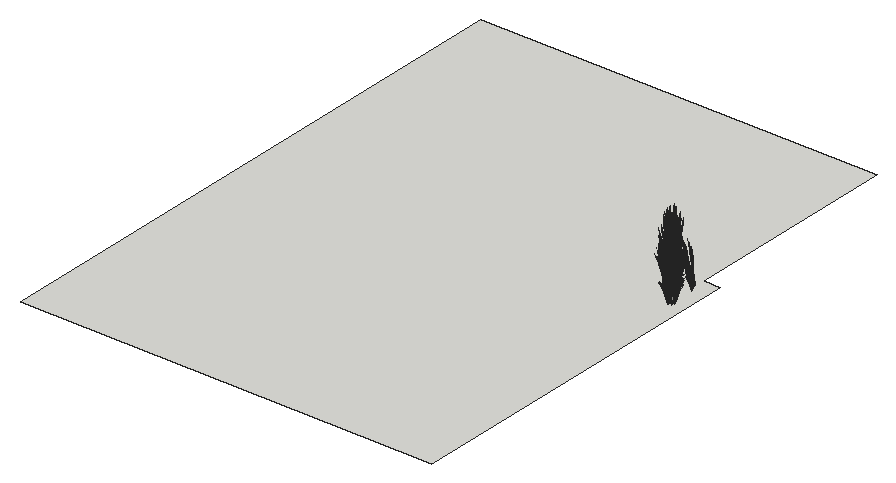
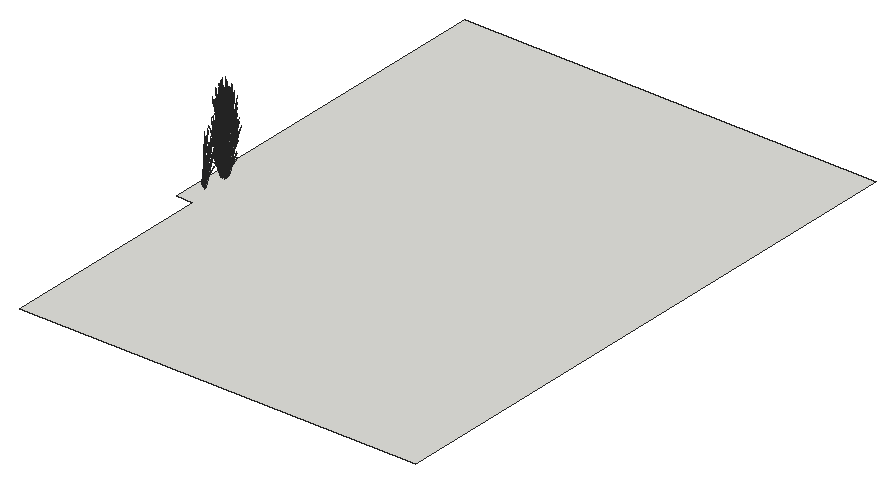
# SketchUp Ruby script. Lengths in inches.
U = 1.inch
M = Sketchup.active_model
def pt(a) = Geom::Point3d.new(a.map { |v| v * U })
def face(e, loops, mat)
  f = e.add_face(loops[0].map { |a| pt(a) })
  loops[1..].each { |l| e.add_face(l.map { |a| pt(a) }).erase! }
  f.material = f.back_material = mat if mat
  f
end
# faces: each face lists its corners as indices into pts; further lists are holes
def faces(e, pts, list, mat = nil) = list.each { |f| face(e, (f[0].is_a?(Array) ? f : [f]).map { |l| l.map { |i| pts[i] } }, mat) }
# xy, xz, yz: faces in a plane at the given z, y or x. An outline is a flat list of corners, or four numbers for a rectangle; further outlines are holes
def ring(l) = l.size == 4 ? [[l[0], l[1]], [l[2], l[1]], [l[2], l[3]], [l[0], l[3]]] : l.each_slice(2).to_a
def flat(e, list, mat, &to3) = list.each { |f| face(e, (f[0].is_a?(Array) ? f : [f]).map { |l| ring(l).map { |u, v| to3.(u, v) } }, mat) }
def xy(e, z, list, mat = nil) = flat(e, list, mat) { |x, y| [x, y, z] }
def xz(e, y, list, mat = nil) = flat(e, list, mat) { |x, z| [x, y, z] }
def yz(e, x, list, mat = nil) = flat(e, list, mat) { |y, z| [x, y, z] }
def lines(e, pts, list) = list.each { |a, b| e.add_line(pt(pts[a]), pt(pts[b])) }
# prism: a flat outline (further loops are holes) pulled along v
def prism(e, loops, v, mat = nil)
  f = face(e, loops, mat); d = Geom::Vector3d.new(v.map { |x| x * U })
  f.pushpull(f.normal.samedirection?(d) ? d.length : -d.length)
end
def box(e, o, s, mat = nil) = prism(e, [[o, [o[0] + s[0], o[1], o[2]], [o[0] + s[0], o[1] + s[1], o[2]], [o[0], o[1] + s[1], o[2]]]], [0, 0, s[2]], mat)
def at(x, y, z, deg = 0) = Geom::Transformation.translation(pt([x, y, z])) * Geom::Transformation.rotation(ORIGIN, Z_AXIS, deg.degrees)
def axes(o, x, y, z) = Geom::Transformation.new([*x, 0, *y, 0, *z, 0, *pt(o).to_a, 1])
def part(name) = M.definitions.add(name)
# library, detail: a bought-in or finely detailed component or shape, given as its bounding box
def library(name, o, s) = part(name).tap { |d| box(d.entities, o, s) }
def detail(e, o, s) = box(e.add_group.entities, o, s)
def put(e, d, t, mat = nil) = e.add_instance(d, t).tap { |i| i.material = mat if mat }
def group(e, t, mat = nil) = e.add_group.tap { |g| g.transformation = t; g.material = mat if mat }.entities
root = M.entities
M.materials.add("LightPink_Translucent").color = [144, 107, 117]
M.materials["LightPink_Translucent"].alpha = 0.75
c1 = part("blade")
p = [[2.15,0.21,22],[0,0.17,0],[0.09,0.45,0],[2.18,0.31,22],[2.29,0.31,22],[0.38,0.45,0],
  [2.48,0.24,33],[2.49,0.24,33],[2.48,0.22,33]]
faces(c1.entities,p,[[0,1,2,3],[4,5,2,3],[6,3,4,7],[8,0,3,6]])
c2 = part("seeds")
p = [[0.3,-0.1,1.38],[-0.01,-0.03,1.59],[-0.01,-0.03,0.03],[0.14,-0.07,-0.07],[0.29,-0.03,3],[0.15,0.01,3.11]]
faces(c2.entities,p,[[0,1,2,3],[1,0,4,5]],"LightPink_Translucent")
c3 = part("blade with seeds")
put(c3.entities,c1,at(0,0,0))
put(c3.entities,c2,axes([2.4,0.25,30.99],[1.5799,-0.05474,1.17369],[-0.12525,1.92788,0.29478],[-0.07173,-0.02425,1.56792]))
xy(root,1398,[[33.57,367.54,339.57,367.54,339.57,634.9,327.57,634.9,327.57,795.7,33.57,795.7]])
put(root,c3,axes([331.43,599.32,1402.73],[0.26007,-0.1585,0.0643],[0.12729,0.28902,0.50621],[-0.02512,-0.1274,0.77189]))
put(root,c3,axes([330.51,599.69,1402.98],[-0.30095,-0.22541,-0.71045],[0.21388,-0.395,0.08574],[-0.10904,-0.13459,1.00501]))
put(root,c3,axes([330.4,599.39,1402.53],[-0.05451,-0.37564,-0.35414],[0.31161,-0.09919,0.4572],[-0.0837,-0.10765,0.87481]))
put(root,c3,axes([330.54,599.36,1402.73],[0.16041,-0.29625,0.0643],[0.22843,0.17248,0.50621],[-0.07385,-0.09498,0.77189]))
put(root,c3,axes([329.92,599.32,1399.49],[-0.03419,0.06144,1.76342],[-0.3455,0.13246,-0.26939],[-0.08346,-0.12049,0.30037]))
put(root,c3,axes([330.49,601.01,1400.1],[-0.14494,-0.47823,-0.69835],[0.41752,-0.17223,-0.18329],[-0.01602,-0.16194,1.54149]))
put(root,c3,axes([329.73,599.94,1401.875],[0.1311,0.08035,1.71376],[-0.27131,0.33708,0.13857],[-0.16909,-0.15206,0.73262]))
put(root,c3,axes([332.43,599.55,1399.49],[-0.05283,-0.03674,1.76342],[-0.13569,-0.41045,-0.26939],[0.09154,-0.11138,0.30037]))
put(root,c3,axes([331.33,599.64,1403.05],[-0.1064,0.35863,0.35414],[-0.31043,-0.1046,-0.4572],[-0.02846,-0.14439,0.87481]))
put(root,c3,axes([330.37,599.7,1402.68],[-0.34827,0.11086,-0.51099],[-0.06092,-0.41983,-0.3958],[-0.09354,-0.12031,0.97773]))
put(root,c3,axes([332.125,599.79,1402.73],[0.25132,0.3182,0.48003],[-0.2669,0.27442,0.3958],[0.04636,-0.14929,0.9933]))
put(root,c3,axes([330.61,599.33,1403.43],[-0.23555,0.44708,-0.13619],[-0.34112,-0.25757,-0.75594],[-0.11858,-0.12631,1.14864]))
put(root,c3,axes([332.22,599.82,1402.73],[0.29004,0.02173,0.0643],[-0.00795,0.32812,0.50621],[0.03035,-0.12569,0.77189]))
put(root,c3,axes([332,600.04,1403.05],[-0.23881,0.24554,0.35414],[-0.22606,-0.28036,-0.4572],[0.0344,-0.14245,0.87481]))
put(root,c3,axes([332.42,600.71,1402.98],[0.18436,-0.36797,-0.71045],[0.32306,0.26151,0.08574],[0.11008,-0.13332,1.00501]))
put(root,c3,axes([330.43,599.63,1400.375],[-0.22066,-0.46731,0],[0.36918,-0.26061,-0.51607],[0.08408,-0.05936,1.63711]))
put(root,c3,axes([332.41,600.53,1402.68],[-0.09067,-0.42583,-0.51099],[0.34336,-0.07449,-0.3958],[0.0984,-0.11438,0.97773]))
put(root,c3,axes([330.92,599.07,1400.13],[-0.2439,0.26754,-0.03893],[-0.22348,-0.29302,-0.17649],[-0.01573,-0.08303,0.58215]))
put(root,c3,axes([329.71,599.2,1402.72],[-0.07594,-0.00329,1.74944],[-0.24177,0.32918,-0.27667],[-0.129,-0.06726,0.14031]))
put(root,c3,axes([332.58,600.84,1403.03],[-0.32648,-0.25715,-0.1216],[0.18809,-0.3724,-0.67495],[0.09224,-0.12945,1.02557]))
put(root,c3,axes([331.23,602.24,1401.33],[0.305,0.18805,1.51261],[-0.29879,0.40513,0.59816],[-0.13384,-0.24012,1.26806]))
put(root,c3,axes([330.59,599.7,1403.05],[0.05451,0.37564,0.35414],[-0.31161,0.09919,-0.4572],[-0.0837,-0.10765,0.87481]))
put(root,c3,axes([329.63,600.94,1400.02],[0,-0.46636,-0.49651],[0.39487,0,0],[0,-0.10622,1.57504]))
put(root,c3,axes([330.73,599.5625,1400.02],[0.33032,-0.23318,-0.49651],[0.19744,0.41812,0],[0.07523,-0.05311,1.57504]))
put(root,c3,axes([332.69,600.37,1400.59],[-0.12609,-0.01381,1.43002],[-0.12917,-0.37055,-0.30754],[0.1549,-0.10482,0.61141]))
put(root,c3,axes([329.65,599.95,1403.09],[0.29147,-0.34417,0.53763],[0.25138,0.3655,0.4433],[-0.13675,-0.06349,1.11249]))
put(root,c3,axes([333.38,600.73,1402.71],[-0.0461,-0.00354,1.77383],[-0.19143,-0.37951,-0.16761],[0.07688,-0.12478,0.31391]))
put(root,c3,axes([331.12,600.52,1400.06],[0.23773,-0.35053,-0.62353],[0.29532,0.31785,-0.16365],[0.09526,-0.08744,1.37633]))
put(root,c3,axes([332.84,599.6875,1400.77],[-0.11756,0.2374,1.1486],[-0.10105,-0.31895,0.84392],[0.09709,-0.07992,0.25299]))
put(root,c3,axes([332.67,600.58,1402.53],[0.30722,-0.06665,-0.35414],[0.08112,0.381,0.4572],[0.08804,-0.10234,0.87481]))
put(root,c3,axes([329.78,599.94,1402.73],[0.01777,-0.35463,0.0643],[0.26836,0.00972,0.50621],[-0.1028,-0.03711,0.77189]))
put(root,c3,axes([330.71,601.13,1400.21],[0.17124,-0.42022,-0.44739],[0.35581,0.20224,0.21531],[0,-0.09687,1.43643]))
put(root,c3,axes([329.68,600.06,1402.53],[-0.20082,-0.29199,-0.35414],[0.2293,-0.2764,0.4572],[-0.1165,-0.04206,0.87481]))
put(root,c3,axes([330.86,600.93,1400.67],[-0.04113,-0.53214,-0.29095],[0.42835,-0.03218,-0.50002],[0.07543,-0.07088,1.59708]))
put(root,c3,axes([329.8,600.95,1400.03],[0.24637,-0.29097,-0.30978],[0.24637,0.29097,0.30978],[0,-0.09372,1.38974]))
put(root,c3,axes([329.7,599.56,1400.13],[-0.10181,0.3808,-0.03893],[-0.31336,-0.11714,-0.17649],[-0.04758,-0.06228,0.58215]))
put(root,c3,axes([332.42,600.8,1403.05],[-0.30722,0.06665,0.35414],[-0.08112,-0.381,-0.4572],[0.08804,-0.10234,0.87481]))
put(root,c3,axes([330.67,601.48,1400.67],[-0.39748,-0.22252,-0.29095],[0.19139,-0.46966,-0.50002],[-0.01249,-0.11531,1.59708]))
put(root,c3,axes([329.53,601.3,1400.375],[-0.44133,0,0],[0,-0.52122,-0.51607],[0,-0.11871,1.63711]))
put(root,c3,axes([329.61,600.37,1400.59],[0.06891,0.12984,1.43002],[-0.15879,0.35293,-0.30754],[-0.16304,-0.08436,0.61141]))
put(root,c3,axes([330.81,599.75,1400.03],[0.32928,0.11539,-0.30978],[-0.08291,0.40636,0.30978],[0.06638,-0.04686,1.38974]))
put(root,c3,axes([329.89,600.25,1402.98],[-0.35281,-0.01123,-0.71045],[0.0237,-0.47284,0.08574],[-0.14947,-0.0499,1.00501]))
put(root,c3,axes([332.7,600.74,1402.73],[0.2423,0.19613,0.0643],[-0.14107,0.2793,0.50621],[0.07768,-0.0903,0.77189]))
put(root,c3,axes([332.63,600.66,1402.73],[0.08753,0.42921,0.48003],[-0.34336,0.07449,0.3958],[0.1012,-0.10094,0.9933]))
put(root,c3,axes([333.55,601.18,1402.72],[0.04898,-0.07104,1.74944],[-0.06269,-0.43574,-0.27667],[0.12289,-0.08262,0.14031]))
put(root,c3,axes([329.875,601.16,1400.33],[-0.32829,0.39208,0.30756],[-0.32849,-0.38796,-0.36492],[-0.01146,-0.11134,1.64885]))
put(root,c3,axes([329.42,599.48,1402.71],[0.02617,0.04654,1.77383],[-0.12614,0.41836,-0.16761],[-0.12775,0.00303,0.31391]))
put(root,c3,axes([330.92,601.34,1400.43],[0.39767,0.22603,0.24065],[-0.19139,0.46966,0.50002],[0,-0.10827,1.60543]))
put(root,c3,axes([330.77,601.98,1400.4375],[0.09355,-0.55261,-0.23429],[0.44354,0.09633,0.51271],[-0.0775,-0.07631,1.5644]))
put(root,c3,axes([329.78,600.35,1402.68],[-0.25628,0.30892,-0.51099],[-0.22444,-0.32634,-0.3958],[-0.13021,-0.047,0.97773]))
put(root,c3,axes([329.97,600.21,1403.05],[0.20082,0.29199,0.35414],[-0.2293,0.2764,-0.4572],[-0.1165,-0.04206,0.87481]))
put(root,c3,axes([329.2,600.76,1400.77],[0.22533,-0.03337,1.1486],[-0.14293,0.29403,0.84392],[-0.11135,-0.04411,0.25299]))
put(root,c3,axes([330.79,601.03,1400.72],[-0.38326,0.02879,0.44739],[-0.03466,-0.47788,-0.21531],[0.06861,-0.04843,1.43643]))
put(root,c3,axes([329.91,600.02,1403.03],[-0.0189,0.47427,-0.1216],[-0.35781,-0.01296,-0.67495],[-0.13781,-0.03295,1.02557]))
put(root,c3,axes([329.8,601.375,1400.48],[0,0.46636,0.49651],[-0.39487,0,0],[0,-0.10622,1.57504]))
put(root,c3,axes([332.59,601.84,1403.03],[-0.17758,-0.42229,-0.1216],[0.31518,-0.20752,-0.67495],[0.13282,-0.05572,1.02557]))
put(root,c3,axes([332.57,601.48,1402.68],[0.09562,-0.42421,-0.51099],[0.32782,0.1454,-0.3958],[0.13199,-0.0389,0.97773]))
put(root,c3,axes([332.06,599.75,1400.375],[0.22066,-0.46731,0],[0.36918,0.26061,-0.51607],[0.08408,0.05936,1.63711]))
put(root,c3,axes([329.46,600.68,1401.875],[0.14639,-0.01056,1.71376],[-0.09712,0.45778,0.13857],[-0.20862,-0.02831,0.73262]))
put(root,c3,axes([330.73,601.75,1400.21],[-0.21202,-0.39143,-0.44739],[0.32115,-0.27564,0.21531],[-0.06861,-0.04843,1.43643]))
put(root,c3,axes([330.78,601.2,1400.36],[0.15345,0.52148,0.45755],[-0.43845,0.18134,0.17955],[0.00536,-0.09582,1.58856]))
put(root,c3,axes([332.92,601.6,1399.98],[-0.22732,0.05597,1.41583],[-0.03618,-0.44548,0.08104],[0.15921,-0.06743,0.80566]))
put(root,c3,axes([333.34,601.2,1400.26],[-0.21881,-0.29821,-0.06488],[0.23965,-0.27324,-0.29416],[0.0679,-0.01924,0.97024]))
put(root,c3,axes([330.7,601.61,1400.72],[-0.17124,0.42022,0.44739],[-0.35581,-0.20224,-0.21531],[0,-0.09687,1.43643]))
put(root,c3,axes([331.33,601.24,1400.21],[0,-0.53961,0],[0.44133,0,0],[0,0,1.79456]))
put(root,c3,axes([331.87,600,1400.48],[-0.33032,-0.23318,0.49651],[0.19744,-0.41812,0],[0.07523,0.05311,1.57504]))
put(root,c3,axes([332.51,601.63,1402.98],[0.31014,-0.20596,-0.71045],[0.17284,0.42397,0.08574],[0.14985,-0.04816,1.00501]))
put(root,c3,axes([330.54,601.9,1400.06],[-0.36714,-0.07646,-0.62353],[0.07747,-0.47163,-0.16365],[-0.10956,-0.05715,1.37633]))
put(root,c3,axes([331.12,600.9,1400.36],[-0.29264,0.42323,0.45755],[-0.34767,-0.3736,0.17955],[0.07055,-0.04224,1.58856]))
put(root,c3,axes([331.44,601.66,1400.3],[-0.32829,-0.4014,-0.06131],[0.32849,-0.40164,0],[-0.01146,-0.01402,1.75571]))
put(root,c3,axes([330.61,600.21,1400.47],[-0.10196,0.46348,0.17642],[-0.3731,-0.13116,0.35086],[0.06445,-0.00226,1.60407]))
put(root,c3,axes([332.47,601.72,1403.05],[-0.29332,-0.1301,0.35414],[0.08555,-0.37955,-0.4572],[0.11809,-0.0348,0.87481]))
put(root,c3,axes([329.4,601.02,1402.73],[0.09971,-0.42522,0.48003],[0.32782,0.1454,0.3958],[-0.12892,0.02555,0.9933]))
put(root,c3,axes([330.46,600.58,1399.59],[-0.3474,0.18671,1.28929],[-0.11057,-0.53572,0.50096],[0.21332,0.00891,1.46642]))
put(root,c3,axes([331.39,600.72,1400.62],[0.06809,-0.4162,0.1448],[0.33266,0.07225,-0.41347],[0.06054,0.04274,1.26744]))
put(root,c3,axes([329.37,600.91,1402.73],[-0.12963,-0.31798,0.0643],[0.23638,-0.15564,0.50621],[-0.1042,0.03071,0.77189]))
put(root,c3,axes([330.82,601.71,1400.36],[0.44609,0.09826,0.45755],[-0.09078,0.55493,0.17955],[-0.06519,-0.05359,1.58856]))
put(root,c3,axes([333.17,601.31,1399.49],[-0.01845,-0.0708,1.76342],[0.12793,-0.41416,-0.26939],[0.12905,-0.00596,0.30037]))
put(root,c3,axes([329.36,601.24,1399.49],[0.00895,0.0735,1.76342],[-0.18044,0.38382,-0.26939],[-0.12817,-0.01935,0.30037]))
put(root,c3,axes([331.25,600.83,1400.72],[-0.21202,-0.39143,0.44739],[0.32115,-0.27564,-0.21531],[0.06861,0.04843,1.43643]))
put(root,c3,axes([330.15,602.62,1400.03],[-0.08291,-0.40636,-0.30978],[0.32928,-0.11539,0.30978],[-0.06638,-0.04686,1.38974]))
put(root,c3,axes([330.58,602.6,1400.47],[0.37926,-0.12378,0.17642],[0.09365,0.46065,0.35086],[-0.03382,-0.06712,1.60407]))
put(root,c3,axes([331.36,600.86,1400.67],[0.35635,-0.30962,-0.29095],[0.23697,0.43749,-0.50002],[0.08792,0.04443,1.59708]))
put(root,c3,axes([332.78,601.67,1402.53],[0.29332,0.1301,-0.35414],[-0.08555,0.37955,0.4572],[0.11809,-0.0348,0.87481]))
put(root,c3,axes([330.0625,602.79,1400.02],[-0.33032,-0.23318,-0.49651],[0.19744,-0.41812,0],[-0.07523,-0.05311,1.57504]))
put(root,c3,axes([332.26,600.03,1400.02],[0.33032,0.23318,-0.49651],[-0.19744,0.41812,0],[0.07523,0.05311,1.57504]))
put(root,c3,axes([329.33,601.07,1402.53],[-0.29332,-0.1301,-0.35414],[0.08555,-0.37955,0.4572],[-0.11809,0.0348,0.87481]))
put(root,c3,axes([331.63,601.36,1400.21],[0.39487,0,0],[0,0.48281,0],[0,0,1.78407]))
put(root,c3,axes([330.96,601.97,1400.67],[-0.35635,0.30962,-0.29095],[-0.23697,-0.43749,-0.50002],[-0.08792,-0.04443,1.59708]))
put(root,c3,axes([331.74,600.23,1400.47],[-0.37926,0.12378,0.17642],[-0.09365,-0.46065,0.35086],[0.03382,0.06712,1.60407]))
put(root,c3,axes([331.98,601.2,1401.875],[-0.14639,0.01056,1.71376],[0.09712,-0.45778,0.13857],[0.20862,0.02831,0.73262]))
put(root,c3,axes([332.17,600.21,1400.03],[0.08291,0.40636,-0.30978],[-0.32928,0.11539,0.30978],[0.06638,0.04686,1.38974]))
put(root,c3,axes([332.73,601.83,1402.73],[0.12963,0.31798,0.0643],[-0.23638,0.15564,0.50621],[0.1042,-0.03071,0.77189]))
put(root,c3,axes([331.5,601.12,1400.38],[-0.44609,-0.09826,0.49198],[0.09078,-0.55493,0.19306],[0.06519,0.05359,1.70813]))
put(root,c3,axes([332.71,601.72,1402.73],[-0.09971,0.42522,0.48003],[-0.32782,-0.1454,0.3958],[0.12892,-0.02555,0.9933]))
put(root,c3,axes([331.15,602.49,1400.2],[-0.11516,-0.40207,0],[0.32884,-0.1408,0],[0,0,1.54371]))
put(root,c3,axes([330.93,602.11,1400.62],[-0.06809,0.4162,0.1448],[-0.33266,-0.07225,-0.41347],[-0.06054,-0.04274,1.26744]))
put(root,c3,axes([329.64,601.03,1403.05],[0.29332,0.1301,0.35414],[-0.08555,0.37955,-0.4572],[-0.11809,0.0348,0.87481]))
put(root,c3,axes([331.58,602.43,1400.18],[0.37054,-0.15823,-0.19198],[0.1302,0.45581,0.00008],[0.0409,-0.01749,1.73897]))
put(root,c3,axes([331.71,602.62,1400.47],[0.10196,-0.46348,0.17642],[0.3731,0.13116,0.35086],[-0.06445,0.00226,1.60407]))
put(root,c3,axes([331.62,601.57,1400.21],[0.24637,0.30123,0],[-0.24637,0.30123,0],[0,0,1.69266]))
put(root,c3,axes([330.22,601.01,1401.34],[0.10032,-0.06746,1.77064],[0.0346,0.47103,0.13857],[-0.2173,0.0625,0.63284]))
put(root,c3,axes([332.29,601.44,1400.47],[-0.2773,-0.3397,0.17642],[0.27945,-0.32949,0.35086],[-0.03063,0.06937,1.60407]))
put(root,c3,axes([331.78,600.93,1400.06],[0.36714,0.07646,-0.62353],[-0.07747,0.47163,-0.16365],[0.10956,0.05715,1.37633]))
put(root,c3,axes([333.4,601.75,1400.77],[-0.21807,0.07699,1.1486],[0.10265,-0.31819,0.84392],[0.11568,0.02177,0.25299]))
put(root,c3,axes([331.07,602.67,1400.2],[-0.35581,-0.20937,0],[0.17124,-0.43505,0],[0,0,1.62707]))
put(root,c3,axes([331.36,602.11,1400.46],[-0.34464,-0.37536,-0.25192],[0.29,-0.42149,0.5513],[-0.0928,0.04391,1.68216]))
put(root,c3,axes([330.45,602.83,1400.48],[0.33032,0.23318,0.49651],[-0.19744,0.41812,0],[-0.07523,-0.05311,1.57504]))
put(root,c3,axes([331.62,601.22,1400.72],[0.17124,-0.42022,0.44739],[0.35581,0.20224,-0.21531],[0,0.09687,1.43643]))
put(root,c3,axes([333.3,603.1,1402.71],[-0.03191,-0.04083,1.77383],[0.06981,-0.43764,-0.16761],[0.12571,-0.02796,0.31391]))
put(root,c3,axes([329.14,601.32,1402.72],[-0.05763,0.06055,1.74944],[0.0049,0.44239,-0.27667],[-0.13211,0.05753,0.14031]))
put(root,c3,axes([331.55,601.46,1400.29],[0,0.53934,-0.05637],[-0.44133,0,0],[0,0.01695,1.79368]))
put(root,c3,axes([329.53,601.26,1402.68],[-0.09562,0.42421,-0.51099],[-0.32782,-0.1454,-0.3958],[-0.13199,0.0389,0.97773]))
put(root,c3,axes([329.51,600.9,1403.03],[0.17758,0.42229,-0.1216],[-0.31518,0.20752,-0.67495],[-0.13282,0.05572,1.02557]))
put(root,c3,axes([331.58,601.08,1400.21],[0.21202,0.39143,-0.44739],[-0.32115,0.27564,0.21531],[0.06861,0.04843,1.43643]))
put(root,c3,axes([333.02,602.73,1401.93],[-0.06755,-0.39203,-0.03492],[0.31928,-0.09013,-0.15832],[0.06667,0.02485,0.52218]))
put(root,c3,axes([330.26,603.08,1400.375],[-0.22066,0.46731,0],[-0.36918,-0.26061,-0.51607],[-0.08408,-0.05936,1.63711]))
put(root,c3,axes([332.19,602.72,1403.03],[0.0189,-0.47427,-0.1216],[0.35781,0.01296,-0.67495],[0.13781,0.03295,1.02557]))
put(root,c3,axes([332.52,601.45,1400.48],[0,-0.46636,0.49651],[0.39487,0,0],[0,0.10622,1.57504]))
put(root,c3,axes([331.53,601.8,1400.72],[0.38326,-0.02879,0.44739],[0.03466,0.47788,-0.21531],[-0.06861,0.04843,1.43643]))
put(root,c3,axes([331.77,601.31,1400.62],[0.32884,-0.136,0.1448],[0.11516,0.38837,-0.41347],[0,0.08547,1.26744]))
put(root,c3,axes([332.14,602.53,1403.05],[-0.20082,-0.29199,0.35414],[0.2293,-0.2764,-0.4572],[0.1165,0.04206,0.87481]))
put(root,c3,axes([331.1875,602.03,1400.21],[-0.38326,0.02879,-0.44739],[-0.03466,-0.47788,0.21531],[-0.06861,0.04843,1.43643]))
put(root,c3,axes([332.99,602.26,1400.59],[-0.085,-0.1147,1.43002],[0.1106,-0.37943,-0.30754],[0.17198,0.0514,0.61141]))
put(root,c3,axes([331.47,602.68,1400.2],[0.35581,0.20937,0],[-0.17124,0.43505,0],[0,0,1.74954]))
put(root,c3,axes([332.5,602.44,1402.72],[0.07571,-0.00789,1.74944],[0.20767,-0.36231,-0.27667],[0.13467,0.04783,0.14031]))
put(root,c3,axes([331.61,603.14,1400.19],[-0.21791,-0.46895,-0.05142],[0.36918,-0.26061,0.51607],[-0.09097,0.04465,1.6363]))
put(root,c3,axes([331.53,602.01,1400.62],[0.26075,0.2802,0.1448],[-0.2175,0.31612,-0.41347],[-0.06054,0.04274,1.26744]))
put(root,c3,axes([329.47,602.08,1402.73],[-0.08753,-0.42921,0.48003],[0.34336,-0.07449,0.3958],[-0.1012,0.10094,0.9933]))
put(root,c3,axes([329.41,602,1402.73],[-0.2423,-0.19613,0.0643],[0.14107,-0.2793,0.50621],[-0.07768,0.0903,0.77189]))
put(root,c3,axes([329.52,601.48,1401.875],[0.12246,-0.09864,1.71376],[0.1031,0.45582,0.13857],[-0.19225,0.10302,0.73262]))
put(root,c3,axes([332.21,602.49,1402.98],[0.35281,0.01123,-0.71045],[-0.0237,0.47284,0.08574],[0.14947,0.0499,1.00501]))
put(root,c3,axes([331.8125,602.87,1400.48],[0.33032,-0.23318,0.49651],[0.19744,0.41812,0],[-0.07523,0.05311,1.57504]))
put(root,c3,axes([331.34,602.5,1400.29],[0.15345,0.53576,-0.06012],[-0.43845,0.18773,0],[0.00536,0.01871,1.72173]))
put(root,c3,axes([331.51,603.08,1400.03],[-0.32928,-0.11539,-0.30978],[0.08291,-0.40636,0.30978],[-0.06638,0.04686,1.38974]))
put(root,c3,axes([329.14,602.26,1400.59],[0.12266,0.03828,1.43002],[0.07906,0.39104,-0.30754],[-0.16661,0.0732,0.61141]))
put(root,c3,axes([329.6875,601.9375,1403.05],[0.30722,-0.06665,0.35414],[0.08112,0.381,-0.4572],[-0.08804,0.10234,0.87481]))
put(root,c3,axes([332.78,601.53,1400.375],[0.44133,0,0],[0,0.52122,-0.51607],[0,0.11871,1.63711]))
put(root,c3,axes([328.5,601.77,1402.71],[0.04504,0.01251,1.77383],[0.13934,0.41205,-0.16761],[-0.0922,0.10815,0.31391]))
put(root,c3,axes([332.61,601.8,1400.2],[-0.44111,-0.00373,-0.04976],[0,-0.52122,0.49943],[-0.01386,0.11865,1.58352]))
put(root,c3,axes([331.65,601.35,1400.67],[0.39748,0.22252,-0.29095],[-0.19139,0.46966,-0.50002],[0.01249,0.11531,1.59708]))
put(root,c3,axes([328.88,603.08,1400.77],[0.14709,-0.21136,1.1486],[0.05804,0.3346,0.84392],[-0.1063,0.05991,0.25299]))
put(root,c3,axes([332.42,602.6875,1402.53],[0.20082,0.29199,-0.35414],[-0.2293,0.2764,0.4572],[0.1165,0.04206,0.87481]))
put(root,c3,axes([332.52,601.875,1400.03],[-0.24637,0.29097,-0.30978],[-0.24637,-0.29097,0.30978],[0,0.09372,1.38974]))
put(root,c3,axes([331.46,601.9,1400.67],[0.04113,0.53214,-0.29095],[-0.42835,0.03218,-0.50002],[-0.07543,0.07088,1.59708]))
put(root,c3,axes([332.32,602.8,1402.73],[-0.01777,0.35463,0.0643],[-0.26836,-0.00972,0.50621],[0.1028,0.03711,0.77189]))
put(root,c3,axes([331.61,601.7,1400.21],[-0.17124,0.42022,-0.44739],[-0.35581,-0.20224,0.21531],[0,0.09687,1.43643]))
put(root,c3,axes([329.43,602.16,1402.53],[-0.30722,0.06665,-0.35414],[-0.08112,-0.381,0.4572],[-0.08804,0.10234,0.87481]))
put(root,c3,axes([332.34,602.6875,1402.73],[-0.26024,0.30729,0.48003],[-0.22444,-0.32634,0.3958],[0.1221,0.05668,0.9933]))
put(root,c3,axes([328.99,603.02,1403.65],[0.31145,0.12449,-0.06488],[-0.0958,0.38314,-0.29416],[-0.05094,0.05817,0.97024]))
put(root,c3,axes([331.2,602.31,1400.06],[-0.23773,0.35053,-0.62353],[-0.29532,-0.31785,-0.16365],[-0.09526,0.08744,1.37633]))
put(root,c3,axes([331.52,603.04,1403.05],[-0.05451,-0.37564,0.35414],[0.31161,-0.09919,-0.4572],[0.0837,0.10765,0.87481]))
put(root,c3,axes([331.62,602.9,1400.33],[0.44186,0.15158,0.30756],[-0.11054,0.54181,-0.36492],[-0.07313,0.06781,1.64885]))
put(root,c3,axes([331.59,603.27,1400.02],[-0.33032,0.23318,-0.49651],[-0.19744,-0.41812,0],[-0.07523,0.05311,1.57504]))
put(root,c3,axes([332.6875,601.89,1400.02],[0,0.46636,-0.49651],[-0.39487,0,0],[0,0.10622,1.57504]))
put(root,c3,axes([331.7,601.9375,1401.875],[-0.1311,-0.08035,1.71376],[0.27131,-0.33708,0.13857],[0.16909,0.15206,0.73262]))
put(root,c3,axes([331.72,600.88,1402.47],[-0.30498,-0.24231,1.38283],[0.32203,-0.37727,0.59665],[0.0984,0.22736,1.33663]))
put(root,c3,axes([329.53,601.9,1403.03],[0.32648,0.25715,-0.1216],[-0.18809,0.3724,-0.67495],[-0.09224,0.12945,1.02557]))
put(root,c3,axes([332.18,602.85,1400.77],[-0.19872,-0.13409,1.1486],[0.2566,-0.13625,0.84392],[0.06921,0.11541,0.25299]))
put(root,c3,axes([331.49,603.24,1403.03],[0.21031,-0.39918,-0.1216],[0.30457,0.22997,-0.67495],[0.10587,0.11278,1.02557]))
put(root,c3,axes([329.97,601.79,1401.875],[0.08815,-0.14329,1.71376],[0.22258,0.38678,0.13857],[-0.15267,0.17614,0.73262]))
put(root,c3,axes([329.6875,602.21,1402.68],[0.09067,0.42583,-0.51099],[-0.34336,0.07449,-0.3958],[-0.0984,0.11438,0.97773]))
put(root,c3,axes([330.1,602.7,1403.05],[0.23881,-0.24554,0.35414],[0.22606,0.28036,-0.4572],[-0.0344,0.14245,0.87481]))
put(root,c3,axes([331.89,603.19,1400.375],[0.22066,0.46731,0],[-0.36918,0.26061,-0.51607],[-0.08408,0.05936,1.63711]))
put(root,c3,axes([331.21,603.57,1402.71],[0.00104,-0.05646,1.77383],[0.30246,-0.2491,-0.16761],[0.10506,0.08891,0.31391]))
put(root,c3,axes([332.24,603.35,1399.49],[0.02571,-0.06733,1.76342],[0.32373,-0.19829,-0.26939],[0.09815,0.10263,0.30037]))
put(root,c3,axes([331.7,601.34,1400.84],[-0.00964,-0.43909,1.41272],[0.43635,0.11382,0.59816],[-0.1032,0.24027,1.3335]))
put(root,c3,axes([331.8125,601.82,1400.09],[0.12941,0.42699,-0.69212],[-0.37279,0.15378,-0.18165],[0.0143,0.14459,1.52773]))
put(root,c3,axes([329.88,602.92,1402.73],[-0.29004,-0.02173,0.0643],[0.00795,-0.32812,0.50621],[-0.03035,0.12569,0.77189]))
put(root,c3,axes([329.27,603.29,1399.49],[0.04734,0.04659,1.76342],[0.08027,0.4317,-0.26939],[-0.10492,0.09206,0.30037]))
put(root,c3,axes([329.98,602.95,1402.73],[-0.25132,-0.3182,0.48003],[0.2669,-0.27442,0.3958],[-0.04636,0.14929,0.9933]))
put(root,c3,axes([331.74,603.04,1402.68],[0.34827,-0.11086,-0.51099],[0.06092,0.41983,-0.3958],[0.09354,0.12031,0.97773]))
put(root,c3,axes([330.77,603.1,1403.05],[0.1064,-0.35863,0.35414],[0.31043,0.1046,-0.4572],[0.02846,0.14439,0.87481]))
put(root,c3,axes([332.22,603.46,1400.67],[-0.22633,-0.01463,1.0506],[0.14947,-0.31064,0.58006],[0.08941,0.11036,0.8241]))
put(root,c3,axes([331.56,603.38,1402.73],[-0.16041,0.29625,0.0643],[-0.22843,-0.17248,0.50621],[0.07385,0.09498,0.77189]))
put(root,c3,axes([331.1875,604.38,1403.65],[0.2439,-0.26754,-0.06488],[0.22348,0.29302,-0.29416],[0.01573,0.08303,0.97024]))
put(root,c3,axes([331.63,603.3,1402.73],[-0.35104,0.10702,0.48003],[-0.06092,-0.41983,0.3958],[0.08256,0.12373,0.9933]))
put(root,c3,axes([329.9,602.14,1401.875],[0.06572,-0.16029,1.71376],[0.27569,0.33172,0.13857],[-0.12437,0.20675,0.73262]))
put(root,c3,axes([331.48,602.71,1400.59],[0.00623,-0.15459,1.43002],[0.29764,-0.17268,-0.30754],[0.09188,0.18503,0.61141]))
put(root,c3,axes([330.67,603.43,1402.73],[-0.26007,0.1585,0.0643],[-0.12729,-0.28902,0.50621],[0.02512,0.1274,0.77189]))
put(root,c3,axes([329.98,603.05,1402.53],[-0.23881,0.24554,-0.35414],[-0.22606,-0.28036,0.4572],[-0.0344,0.14245,0.87481]))
put(root,c3,axes([329.15,602.97,1402.72],[-0.00877,0.09229,1.74944],[0.24897,0.32105,-0.27667],[-0.06518,0.15182,0.14031]))
put(root,c3,axes([329.95,602.76,1403.4],[0.3879,0.02311,-0.13498],[-0.0106,0.43749,-0.74919],[-0.02694,0.1685,1.13838]))
put(root,c3,axes([330.67,603.25,1403.03],[0.34538,-0.21713,-0.1216],[0.16972,0.38536,-0.67495],[0.04557,0.16239,1.02557]))
put(root,c3,axes([330.77,603.4,1403.0625],[-0.34777,-0.12192,0.53283],[0.11892,-0.40083,0.43934],[0.0209,0.15763,1.10256]))
put(root,c3,axes([330.13,604,1400.77],[-0.00913,-0.2773,1.1486],[0.22824,0.19778,0.84392],[-0.04489,0.13217,0.25299]))
put(root,c3,axes([330.73,603.34,1399.49],[0.05712,-0.02538,1.76342],[0.34359,0.13968,-0.26939],[0.01005,0.15742,0.30037]))
put(root,c3,axes([330.21,602.93,1403],[0.25266,0.31335,-0.5672],[-0.2669,0.27442,-0.43934],[-0.03844,0.15921,1.08528]))
put(root,c3,axes([329.9375,603.4,1400.82],[0.32063,-0.08258,0.06507],[0.07371,0.33271,-0.86304],[-0.02033,0.16842,0.7736]))
put(root,c3,axes([330.96,603.23,1402.68],[0.34695,0.11691,-0.51099],[-0.11892,0.40083,-0.3958],[0.03181,0.16138,0.97773]))
put(root,c3,axes([331.16,602.41,1401.875],[-0.08068,-0.14973,1.71376],[0.3728,-0.12606,0.13857],[0.08426,0.23506,0.73262]))
put(root,c3,axes([330.8,603.48,1402.53],[-0.1064,0.35863,-0.35414],[-0.31043,-0.1046,0.4572],[0.02846,0.14439,0.87481]))
put(root,c3,axes([330.13,602.79,1403.34],[-0.00918,0.43138,-0.7886],[-0.38672,-0.02897,0.09517],[-0.04081,0.18275,1.11556]))
put(root,c3,axes([329.125,603.92,1402.71],[0.04004,-0.02816,1.77383],[0.33095,0.18728,-0.16761],[-0.00778,0.15594,0.31391]))
put(root,c3,axes([330.5,602.48,1401.875],[-0.00864,-0.17899,1.71376],[0.37441,0.11874,0.13857],[-0.02316,0.25508,0.73262]))
put(root,c3,axes([330.84,603.16,1402.98],[0.16845,0.3792,-0.71045],[-0.34676,0.21133,0.08574],[0.03939,0.18322,1.00501]))
put(root,c3,axes([329.86,603.75,1400.59],[0.11138,-0.07357,1.43002],[0.27499,0.22183,-0.30754],[-0.08185,0.19194,0.61141]))
put(root,c3,axes([330.58,604.11,1402.72],[0.04474,0.0751,1.74944],[0.36104,0.0295,-0.27667],[0.03631,0.16562,0.14031]))
put(root,c3,axes([330.01,603.39,1401.36],[0.00775,-0.24075,1.54345],[0.34877,0.12716,0.21329],[-0.03022,0.25658,0.72882]))
put(root,c3,axes([330.27,620.6,1401.875],[0.08068,0.14973,1.71376],[-0.3728,0.12606,0.13857],[-0.08426,-0.23506,0.73262]))
put(root,c3,axes([330.89,619.61,1402.72],[-0.05398,-0.06539,1.74944],[-0.36026,0.04145,-0.27667],[-0.0575,-0.15639,0.14031]))
put(root,c3,axes([331.72,620.39,1400.59],[-0.10032,0.0944,1.43002],[-0.30046,-0.16522,-0.30754],[0.05569,-0.20547,0.61141]))
put(root,c3,axes([331.27,620.72,1402.98],[-0.16845,-0.3792,-0.71045],[0.34676,-0.21133,0.08574],[-0.03939,-0.18322,1.00501]))
put(root,c3,axes([330.17,620.21,1400.59],[-0.02137,0.15256,1.43002],[-0.31245,0.12771,-0.30754],[-0.07303,-0.19719,0.61141]))
put(root,c3,axes([330.98,619.875,1399.49],[-0.0592,0.0168,1.76342],[-0.32738,-0.18913,-0.26939],[0.00549,-0.15776,0.30037]))
put(root,c3,axes([331.97,621.09,1402.98],[0.00918,-0.43138,-0.71045],[0.38672,0.02897,0.08574],[0.04081,-0.18275,1.00501]))
put(root,c3,axes([332.51,620.41,1402.72],[-0.00341,-0.09282,1.74944],[-0.28775,-0.26825,-0.27667],[0.04449,-0.16261,0.14031]))
put(root,c3,axes([331.3,620.39,1402.53],[0.1064,-0.35863,-0.35414],[0.31043,0.1046,0.4572],[-0.02846,-0.14439,0.87481]))
put(root,c3,axes([331.53,620.87,1401.875],[-0.06572,0.16029,1.71376],[-0.27569,-0.33172,0.13857],[0.12437,-0.20675,0.73262]))
